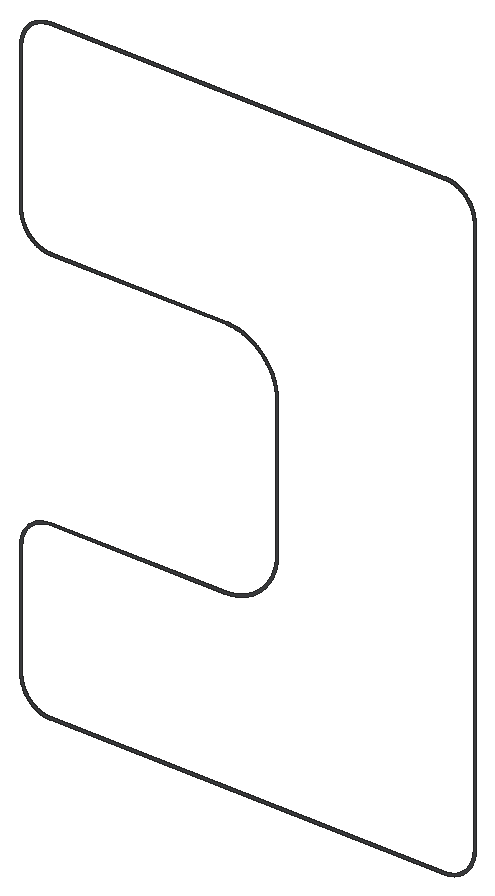
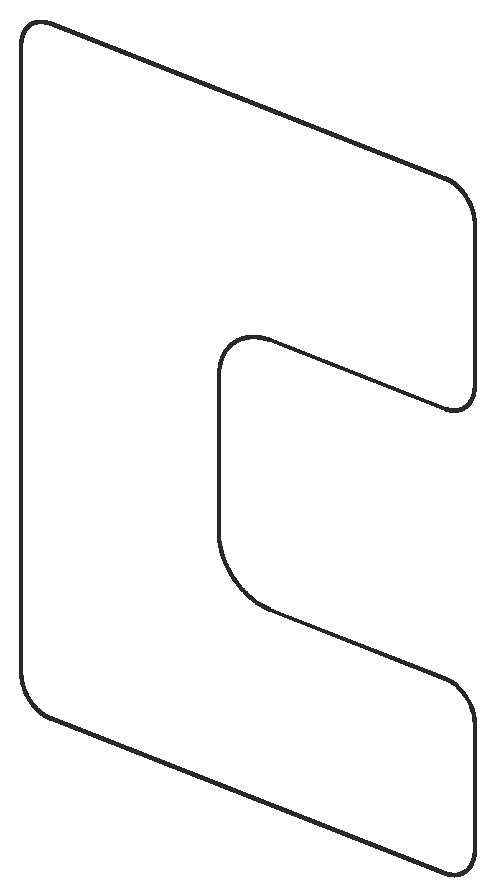
# SketchUp Ruby script. Lengths in inches.
U = 1.inch
M = Sketchup.active_model
def pt(a) = Geom::Point3d.new(a.map { |v| v * U })
def face(e, loops, mat)
  f = e.add_face(loops[0].map { |a| pt(a) })
  loops[1..].each { |l| e.add_face(l.map { |a| pt(a) }).erase! }
  f.material = f.back_material = mat if mat
  f
end
# faces: each face lists its corners as indices into pts; further lists are holes
def faces(e, pts, list, mat = nil) = list.each { |f| face(e, (f[0].is_a?(Array) ? f : [f]).map { |l| l.map { |i| pts[i] } }, mat) }
# xy, xz, yz: faces in a plane at the given z, y or x. An outline is a flat list of corners, or four numbers for a rectangle; further outlines are holes
def ring(l) = l.size == 4 ? [[l[0], l[1]], [l[2], l[1]], [l[2], l[3]], [l[0], l[3]]] : l.each_slice(2).to_a
def flat(e, list, mat, &to3) = list.each { |f| face(e, (f[0].is_a?(Array) ? f : [f]).map { |l| ring(l).map { |u, v| to3.(u, v) } }, mat) }
def xy(e, z, list, mat = nil) = flat(e, list, mat) { |x, y| [x, y, z] }
def xz(e, y, list, mat = nil) = flat(e, list, mat) { |x, z| [x, y, z] }
def yz(e, x, list, mat = nil) = flat(e, list, mat) { |y, z| [x, y, z] }
def lines(e, pts, list) = list.each { |a, b| e.add_line(pt(pts[a]), pt(pts[b])) }
# prism: a flat outline (further loops are holes) pulled along v
def prism(e, loops, v, mat = nil)
  f = face(e, loops, mat); d = Geom::Vector3d.new(v.map { |x| x * U })
  f.pushpull(f.normal.samedirection?(d) ? d.length : -d.length)
end
def box(e, o, s, mat = nil) = prism(e, [[o, [o[0] + s[0], o[1], o[2]], [o[0] + s[0], o[1] + s[1], o[2]], [o[0], o[1] + s[1], o[2]]]], [0, 0, s[2]], mat)
def at(x, y, z, deg = 0) = Geom::Transformation.translation(pt([x, y, z])) * Geom::Transformation.rotation(ORIGIN, Z_AXIS, deg.degrees)
def axes(o, x, y, z) = Geom::Transformation.new([*x, 0, *y, 0, *z, 0, *pt(o).to_a, 1])
def part(name) = M.definitions.add(name)
# library, detail: a bought-in or finely detailed component or shape, given as its bounding box
def library(name, o, s) = part(name).tap { |d| box(d.entities, o, s) }
def detail(e, o, s) = box(e.add_group.entities, o, s)
def put(e, d, t, mat = nil) = e.add_instance(d, t).tap { |i| i.material = mat if mat }
def group(e, t, mat = nil) = e.add_group.tap { |g| g.transformation = t; g.material = mat if mat }.entities
root = M.entities
M.materials.add("1432 AP 8245 TAR ROAD").color = [71, 72, 75]
xz(root,96.87,[[[278.68,171.29,537.32,171.29,537.48,171.3,537.64,171.3,537.8,171.31,537.97,171.31,538.125,171.32,538.29,171.33,538.45,171.34,538.61,171.36,538.93,171.38,539.25,171.42,539.41,171.43,539.73,171.47,539.89,171.5,540.21,171.54,540.37,171.57,540.52,171.6,540.68,171.625,540.84,171.66,541,171.6875,541.16,171.72,541.31,171.75,541.47,171.79,541.63,171.82,541.79,171.86,541.94,171.9,542.1,171.9375,542.25,171.98,542.41,172.02,542.56,172.0625,542.72,172.11,542.875,172.15,543.03,172.2,543.33,172.3,543.49,172.35,543.94,172.5,544.1,172.56,544.25,172.62,544.4,172.67,544.85,172.85,544.99,172.91,545.14,172.98,545.29,173.04,545.4375,173.11,545.58,173.18,545.73,173.24,545.875,173.3125,546.02,173.38,546.16,173.45,546.31,173.53,546.59,173.67,546.73,173.75,547.02,173.91,547.44,174.15,547.57,174.23,547.71,174.3125,547.85,174.4,547.98,174.48,548.12,174.57,548.25,174.66,548.39,174.75,548.52,174.84,548.66,174.93,548.92,175.11,549.05,175.21,549.18,175.3,549.31,175.4,549.4375,175.5,549.56,175.59,549.82,175.79,549.94,175.89,550.07,176,550.19,176.1,550.3125,176.2,550.4375,176.31,550.56,176.41,550.92,176.74,551.03,176.85,551.27,177.07,551.61,177.41,551.72,177.53,551.83,177.64,551.94,177.76,552.05,177.875,552.16,178,552.27,178.11,552.38,178.24,552.48,178.36,552.59,178.48,552.69,178.6,552.8,178.72,552.9,178.85,553,178.97,553.3,179.36,553.39,179.48,553.49,179.61,553.58,179.74,553.68,179.875,553.77,180,553.86,180.14,553.96,180.27,554.05,180.4,554.13,180.54,554.22,180.67,554.31,180.81,554.39,180.94,554.48,181.08,554.5625,181.22,554.65,181.36,554.89,181.78,554.96,181.92,555.12,182.2,555.19,182.34,555.27,182.49,555.41,182.77,555.48,182.92,555.55,183.0625,555.62,183.21,555.68,183.36,555.75,183.5,555.8125,183.65,555.88,183.8,556.18,184.55,556.23,184.7,556.29,184.85,556.39,185.15,556.45,185.3,556.5,185.46,556.55,185.61,556.59,185.76,556.64,185.92,556.6875,186.07,556.73,186.23,556.77,186.38,556.82,186.54,556.86,186.69,556.9,186.85,556.93,187.01,556.97,187.16,557.01,187.32,557.04,187.48,557.07,187.63,557.11,187.79,557.17,188.11,557.19,188.27,557.25,188.59,557.27,188.74,557.3,188.9,557.32,189.0625,557.34,189.22,557.36,189.38,557.39,189.7,557.41,189.86,557.42,190.02,557.4375,190.18,557.45,190.34,557.46,190.5,557.47,190.67,557.48,190.83,557.48,190.99,557.49,191.15,557.49,191.31,557.5,191.47,557.5,561.11,557.49,561.28,557.49,561.4375,557.48,561.6,557.48,561.76,557.45,562.24,557.4375,562.4,557.42,562.5625,557.41,562.72,557.39,562.88,557.36,563.2,557.3,563.68,557.27,563.84,557.25,564,557.19,564.32,557.17,564.48,557.14,564.63,557.11,564.79,557.07,564.95,557.04,565.11,557.01,565.26,556.93,565.58,556.9,565.73,556.82,566.05,556.77,566.2,556.73,566.36,556.6875,566.51,556.64,566.67,556.59,566.82,556.55,566.97,556.45,567.28,556.39,567.43,556.34,567.58,556.29,567.74,556.23,567.89,556.18,568.04,556.12,568.1875,556.06,568.34,555.88,568.79,555.8125,568.93,555.75,569.08,555.68,569.23,555.62,569.375,555.55,569.52,555.48,569.67,555.41,569.8125,555.34,569.96,555.27,570.1,555.19,570.24,555.12,570.38,555.04,570.53,554.96,570.67,554.89,570.81,554.65,571.23,554.5625,571.37,554.48,571.5,554.39,571.64,554.31,571.78,554.22,571.91,554.13,572.05,554.05,572.18,553.96,572.31,553.86,572.45,553.68,572.71,553.58,572.84,553.49,572.97,553.39,573.1,553.3,573.23,553.2,573.36,553.1,573.48,553,573.61,552.9,573.73,552.8,573.86,552.69,573.98,552.59,574.11,552.48,574.23,552.38,574.35,551.94,574.83,551.83,574.94,551.72,575.06,551.61,575.17,551.5,575.29,551.38,575.4,551.27,575.51,551.03,575.74,550.92,575.85,550.8,575.95,550.68,576.0625,550.56,576.17,550.4375,576.28,550.3125,576.38,550.19,576.48,550.07,576.59,549.94,576.69,549.82,576.79,549.56,576.99,549.4375,577.09,549.31,577.1875,549.18,577.28,548.92,577.47,548.79,577.5625,548.66,577.66,548.52,577.75,548.39,577.84,548.25,577.93,548.12,578.01,547.98,578.1,547.85,578.1875,547.71,578.27,547.57,578.35,547.44,578.4375,547.3,578.52,547.02,578.68,546.875,578.76,546.73,578.83,546.59,578.91,546.45,578.98,546.31,579.06,546.16,579.13,546.02,579.2,545.73,579.34,545.58,579.41,545.4375,579.48,545.29,579.54,545.14,579.61,544.99,579.67,544.85,579.73,544.25,579.97,544.1,580.02,543.94,580.08,543.79,580.13,543.64,580.1875,543.49,580.24,543.33,580.29,543.03,580.39,542.875,580.43,542.72,580.48,542.56,580.52,542.41,580.57,542.25,580.61,542.1,580.65,541.94,580.6875,541.79,580.73,541.63,580.76,541.47,580.8,541.31,580.83,541.16,580.87,540.52,580.99,540.37,581.01,540.21,581.04,540.05,581.0625,539.89,581.09,539.09,581.19,538.93,581.2,538.77,581.22,538.29,581.25,538.125,581.26,537.97,581.27,537.8,581.28,537.64,581.28,537.48,581.29,278.52,581.29,278.36,581.28,278.2,581.28,278.03,581.27,277.875,581.26,277.71,581.25,277.23,581.22,277.07,581.2,276.91,581.19,276.11,581.09,275.95,581.0625,275.79,581.04,275.63,581.01,275.48,580.99,274.84,580.87,274.69,580.83,274.53,580.8,274.37,580.76,274.21,580.73,274.06,580.6875,273.9,580.65,273.75,580.61,273.59,580.57,273.44,580.52,273.28,580.48,273.125,580.43,272.97,580.39,272.67,580.29,272.51,580.24,272.36,580.1875,272.21,580.13,272.06,580.08,271.9,580.02,271.75,579.97,271.15,579.73,271.01,579.67,270.86,579.61,270.71,579.54,270.5625,579.48,270.42,579.41,270.27,579.34,269.98,579.2,269.84,579.13,269.69,579.06,269.55,578.98,269.41,578.91,269.27,578.83,269.125,578.76,268.98,578.68,268.7,578.52,268.56,578.4375,268.43,578.35,268.29,578.27,268.15,578.1875,268.02,578.1,267.88,578.01,267.75,577.93,267.61,577.84,267.48,577.75,267.34,577.66,267.21,577.5625,267.08,577.47,266.82,577.28,266.69,577.1875,266.5625,577.09,266.44,576.99,266.18,576.79,266.06,576.69,265.93,576.59,265.81,576.48,265.6875,576.38,265.5625,576.28,265.44,576.17,265.32,576.0625,265.2,575.95,265.08,575.85,264.97,575.74,264.73,575.51,264.62,575.4,264.5,575.29,264.39,575.17,264.28,575.06,264.17,574.94,264.06,574.83,263.62,574.35,263.52,574.23,263.41,574.11,263.31,573.98,263.2,573.86,263.1,573.73,263,573.61,262.9,573.48,262.8,573.36,262.7,573.23,262.61,573.1,262.51,572.97,262.42,572.84,262.32,572.71,262.14,572.45,262.04,572.31,261.95,572.18,261.87,572.05,261.78,571.91,261.69,571.78,261.61,571.64,261.52,571.5,261.4375,571.37,261.35,571.23,261.11,570.81,261.04,570.67,260.96,570.53,260.88,570.38,260.81,570.24,260.73,570.1,260.66,569.96,260.59,569.8125,260.52,569.67,260.45,569.52,260.38,569.375,260.32,569.23,260.25,569.08,260.1875,568.93,260.12,568.79,259.94,568.34,259.88,568.1875,259.82,568.04,259.77,567.89,259.71,567.74,259.66,567.58,259.61,567.43,259.55,567.28,259.45,566.97,259.41,566.82,259.36,566.67,259.3125,566.51,259.27,566.36,259.23,566.2,259.18,566.05,259.1,565.73,259.07,565.58,258.99,565.26,258.96,565.11,258.93,564.95,258.89,564.79,258.86,564.63,258.83,564.48,258.81,564.32,258.75,564,258.73,563.84,258.7,563.68,258.64,563.2,258.61,562.88,258.59,562.72,258.58,562.5625,258.5625,562.4,258.55,562.24,258.52,561.76,258.52,561.6,258.51,561.4375,258.51,561.28,258.5,561.11,258.5,464.47,258.51,464.31,258.51,464.15,258.52,463.99,258.52,463.83,258.53,463.67,258.54,463.5,258.55,463.34,258.5625,463.18,258.58,463.02,258.59,462.86,258.61,462.7,258.64,462.38,258.66,462.22,258.68,462.0625,258.7,461.9,258.73,461.74,258.75,461.59,258.81,461.27,258.83,461.11,258.89,460.79,258.93,460.63,258.96,460.48,258.99,460.32,259.03,460.16,259.07,460.01,259.1,459.85,259.14,459.69,259.18,459.54,259.23,459.38,259.27,459.23,259.3125,459.07,259.36,458.92,259.41,458.76,259.45,458.61,259.5,458.46,259.55,458.3,259.61,458.15,259.71,457.85,259.77,457.7,259.82,457.55,260.12,456.8,260.1875,456.65,260.25,456.5,260.32,456.36,260.38,456.21,260.45,456.0625,260.52,455.92,260.59,455.77,260.73,455.49,260.81,455.34,260.88,455.2,261.04,454.92,261.11,454.78,261.35,454.36,261.4375,454.22,261.52,454.08,261.61,453.94,261.69,453.81,261.78,453.67,261.87,453.54,261.95,453.4,262.04,453.27,262.14,453.14,262.23,453,262.32,452.875,262.42,452.74,262.51,452.61,262.61,452.48,262.7,452.36,263,451.97,263.1,451.85,263.2,451.72,263.31,451.6,263.41,451.48,263.52,451.36,263.62,451.24,263.73,451.11,263.84,451,263.95,450.875,264.06,450.76,264.17,450.64,264.28,450.53,264.39,450.41,264.73,450.07,264.97,449.85,265.08,449.74,265.44,449.41,265.5625,449.31,265.6875,449.2,265.81,449.1,265.93,449,266.06,448.89,266.18,448.79,266.44,448.59,266.5625,448.5,266.69,448.4,266.82,448.3,266.95,448.21,267.08,448.11,267.34,447.93,267.48,447.84,267.61,447.75,267.75,447.66,267.88,447.57,268.02,447.48,268.15,447.4,268.29,447.3125,268.43,447.23,268.56,447.15,268.98,446.91,269.27,446.75,269.41,446.67,269.69,446.53,269.84,446.45,269.98,446.38,270.125,446.3125,270.27,446.24,270.42,446.18,270.5625,446.11,270.71,446.04,270.86,445.98,271.01,445.91,271.15,445.85,271.6,445.67,271.75,445.62,271.9,445.56,272.06,445.5,272.51,445.35,272.67,445.3,272.97,445.2,273.125,445.15,273.28,445.11,273.44,445.0625,273.59,445.02,273.75,444.98,273.9,444.9375,274.06,444.9,274.21,444.86,274.37,444.82,274.53,444.79,274.69,444.75,274.84,444.72,275,444.6875,275.16,444.66,275.32,444.625,275.48,444.6,275.63,444.57,275.79,444.54,276.11,444.5,276.27,444.47,276.59,444.43,276.75,444.42,277.07,444.38,277.39,444.36,277.55,444.34,277.71,444.33,277.875,444.32,278.03,444.31,278.2,444.31,278.36,444.3,278.52,444.3,278.68,444.29,393.4375,444.29,393.875,444.28,394.32,444.27,394.75,444.25,395.19,444.22,395.63,444.1875,396.07,444.15,396.5,444.11,396.9375,444.06,397.37,444.01,397.81,443.95,398.67,443.81,399.1,443.73,399.54,443.65,399.97,443.56,400.39,443.47,400.82,443.37,401.25,443.26,401.67,443.15,402.93,442.79,403.77,442.51,404.18,442.37,404.59,442.22,405.01,442.07,405.41,441.91,405.82,441.74,406.22,441.57,406.625,441.4,407.03,441.21,407.42,441.03,407.82,440.84,408.21,440.64,408.6,440.4375,408.98,440.23,409.37,440.02,410.13,439.58,410.5,439.36,411.25,438.89,411.61,438.65,412.33,438.15,412.69,437.89,413.39,437.37,413.74,437.1,414.08,436.83,414.76,436.27,415.09,435.98,415.42,435.6875,415.74,435.39,416.06,435.09,416.375,434.79,417,434.17,417.9,433.21,418.1875,432.88,418.47,432.55,418.76,432.21,419.03,431.875,419.31,431.53,419.58,431.1875,419.84,430.84,420.1,430.48,420.36,430.125,420.61,429.77,420.85,429.4,421.1,429.04,421.33,428.67,421.5625,428.3,421.79,427.92,422.23,427.16,422.44,426.78,422.65,426.39,423.05,425.61,423.24,425.21,423.42,424.82,423.78,424.02,423.95,423.61,424.12,423.21,424.27,422.8,424.43,422.39,424.58,421.97,424.72,421.56,424.86,421.14,424.99,420.73,425.12,420.31,425.24,419.89,425.36,419.46,425.47,419.04,425.57,418.61,425.67,418.19,425.77,417.76,425.86,417.33,425.9375,416.9,426.02,416.47,426.09,416.03,426.15,415.6,426.21,415.16,426.27,414.73,426.32,414.29,426.36,413.86,426.4,413.42,426.43,412.98,426.45,412.55,426.49,411.67,426.5,411.23,426.5,320.35,426.49,319.92,426.43,318.6,426.4,318.16,426.36,317.73,426.32,317.29,426.27,316.85,426.15,315.99,426.09,315.55,426.02,315.12,425.9375,314.6875,425.86,314.26,425.77,313.83,425.57,312.97,425.47,312.55,425.36,312.12,425.12,311.28,424.86,310.44,424.72,310.02,424.58,309.61,424.43,309.2,424.27,308.79,424.12,308.38,423.95,307.97,423.78,307.57,423.24,306.37,423.05,305.98,422.85,305.58,422.65,305.19,422.44,304.81,422.23,304.42,421.79,303.66,421.5625,303.29,421.33,302.92,421.1,302.55,420.85,302.18,420.61,301.82,420.36,301.46,420.1,301.1,419.58,300.4,419.31,300.05,419.03,299.71,418.76,299.37,418.47,299.04,418.1875,298.7,417.9,298.375,417.6,298.05,417.3,297.73,417,297.42,416.6875,297.1,416.375,296.8,416.06,296.49,415.74,296.19,415.42,295.9,414.76,295.32,413.74,294.48,413.39,294.21,412.69,293.69,412.33,293.43,411.97,293.18,411.61,292.9375,411.25,292.7,410.875,292.46,410.5,292.23,410.13,292,409.75,291.78,409.37,291.5625,408.98,291.35,408.6,291.14,408.21,290.94,407.82,290.75,407.42,290.56,407.03,290.37,406.625,290.1875,406.22,290.01,405.82,289.84,405.41,289.68,405.01,289.52,404.59,289.36,404.18,289.21,403.77,289.07,403.35,288.93,402.51,288.67,401.67,288.43,401.25,288.32,400.39,288.12,399.97,288.02,399.54,287.9375,399.1,287.85,398.67,287.78,398.24,287.7,397.81,287.64,397.37,287.58,396.9375,287.52,396.5,287.48,396.07,287.43,395.63,287.4,395.19,287.36,394.75,287.34,394.32,287.32,393.875,287.3,393.4375,287.29,279,287.29,276.32,287.12,273.69,286.59,271.15,285.73,268.75,284.55,266.52,283.06,264.5,281.29,262.74,279.27,261.25,277.04,260.06,274.64,259.2,272.1,258.68,269.47,258.5,266.79,258.5,191.47,258.51,191.31,258.51,191.15,258.52,190.99,258.52,190.83,258.53,190.67,258.54,190.5,258.55,190.34,258.5625,190.18,258.58,190.02,258.59,189.86,258.61,189.7,258.64,189.38,258.66,189.22,258.68,189.0625,258.7,188.9,258.73,188.74,258.75,188.59,258.81,188.27,258.83,188.11,258.89,187.79,258.93,187.63,258.96,187.48,258.99,187.32,259.03,187.16,259.07,187.01,259.1,186.85,259.14,186.69,259.18,186.54,259.23,186.38,259.27,186.23,259.3125,186.07,259.36,185.92,259.41,185.76,259.45,185.61,259.5,185.46,259.55,185.3,259.61,185.15,259.71,184.85,259.77,184.7,259.82,184.55,260.12,183.8,260.1875,183.65,260.25,183.5,260.32,183.36,260.38,183.21,260.45,183.0625,260.52,182.92,260.59,182.77,260.73,182.49,260.81,182.34,260.88,182.2,261.04,181.92,261.11,181.78,261.35,181.36,261.4375,181.22,261.52,181.08,261.61,180.94,261.69,180.81,261.78,180.67,261.87,180.54,261.95,180.4,262.04,180.27,262.14,180.14,262.23,180,262.32,179.875,262.42,179.74,262.51,179.61,262.61,179.48,262.7,179.36,263,178.97,263.1,178.85,263.2,178.72,263.31,178.6,263.41,178.48,263.52,178.36,263.62,178.24,263.73,178.11,263.84,178,263.95,177.875,264.06,177.76,264.17,177.64,264.28,177.53,264.39,177.41,264.73,177.07,264.97,176.85,265.08,176.74,265.44,176.41,265.5625,176.31,265.6875,176.2,265.81,176.1,265.93,176,266.06,175.89,266.18,175.79,266.44,175.59,266.5625,175.5,266.69,175.4,266.82,175.3,266.95,175.21,267.08,175.11,267.34,174.93,267.48,174.84,267.61,174.75,267.75,174.66,267.88,174.57,268.02,174.48,268.15,174.4,268.29,174.3125,268.43,174.23,268.56,174.15,268.98,173.91,269.27,173.75,269.41,173.67,269.69,173.53,269.84,173.45,269.98,173.38,270.125,173.3125,270.27,173.24,270.42,173.18,270.5625,173.11,270.71,173.04,270.86,172.98,271.01,172.91,271.15,172.85,271.6,172.67,271.75,172.62,271.9,172.56,272.06,172.5,272.51,172.35,272.67,172.3,272.97,172.2,273.125,172.15,273.28,172.11,273.44,172.0625,273.59,172.02,273.75,171.98,273.9,171.9375,274.06,171.9,274.21,171.86,274.37,171.82,274.53,171.79,274.69,171.75,274.84,171.72,275,171.6875,275.16,171.66,275.32,171.625,275.48,171.6,275.63,171.57,275.79,171.54,276.11,171.5,276.27,171.47,276.59,171.43,276.75,171.42,277.07,171.38,277.39,171.36,277.55,171.34,277.71,171.33,277.875,171.32,278.03,171.31,278.2,171.31,278.36,171.3,278.52,171.3],[278.7,172.79,278.55,172.8,278.4,172.8,278.25,172.81,278.1,172.8125,277.96,172.82,277.36,172.86,277.21,172.875,277.0625,172.89,276.92,172.91,276.77,172.92,276.32,172.98,276.18,173,276.03,173.03,275.73,173.07,275.59,173.1,275.29,173.16,275.15,173.1875,275,173.22,274.86,173.25,274.71,173.28,274.56,173.32,274.42,173.35,274.27,173.39,273.99,173.47,273.84,173.51,273.56,173.59,273.41,173.63,273.27,173.68,273.13,173.72,272.85,173.82,272.7,173.87,272.5625,173.92,272.42,173.97,272.14,174.07,272.01,174.125,271.87,174.18,271.59,174.3,271.45,174.35,271.32,174.41,271.18,174.48,271.05,174.54,270.91,174.6,270.78,174.66,270.64,174.73,270.51,174.8,270.375,174.86,270.24,174.93,269.72,175.21,269.59,175.29,269.46,175.36,269.33,175.4375,269.2,175.51,269.07,175.59,268.95,175.67,268.69,175.83,268.57,175.91,268.44,175.99,268.32,176.08,268.2,176.16,268.07,176.25,267.95,176.33,267.59,176.6,267.47,176.6875,267.35,176.78,267.24,176.87,267.12,176.96,267,177.06,266.89,177.15,266.77,177.25,266.66,177.34,266.44,177.54,266.32,177.64,265.99,177.94,265.78,178.15,265.67,178.25,265.46,178.46,265.36,178.57,265.25,178.68,265.15,178.79,265.05,178.89,264.95,179,264.85,179.12,264.55,179.45,264.46,179.57,264.36,179.68,264.27,179.8,264.17,179.91,263.9,180.27,263.81,180.38,263.72,180.5,263.54,180.75,263.46,180.87,263.37,180.99,263.29,181.11,263.2,181.24,263.12,181.36,263.04,181.49,262.96,181.61,262.88,181.74,262.8,181.86,262.72,181.99,262.65,182.12,262.57,182.25,262.5,182.38,262.42,182.51,262.14,183.03,262.07,183.17,262,183.3,261.9375,183.43,261.87,183.57,261.81,183.7,261.75,183.84,261.68,183.97,261.62,184.11,261.5625,184.25,261.5,184.38,261.45,184.52,261.33,184.8,261.28,184.9375,261.23,185.08,261.17,185.22,261.125,185.36,261.07,185.5,261.02,185.64,260.98,185.78,260.93,185.92,260.88,186.0625,260.84,186.21,260.8,186.35,260.75,186.49,260.71,186.63,260.67,186.78,260.63,186.92,260.6,187.07,260.56,187.21,260.52,187.36,260.49,187.5,260.46,187.65,260.43,187.79,260.39,187.9375,260.37,188.09,260.34,188.23,260.28,188.53,260.26,188.67,260.23,188.82,260.21,188.97,260.19,189.11,260.11,189.71,260.1,189.86,260.08,190,260.01,191.05,260.01,191.34,260,191.49,260,266.79,260.16,269.27,260.65,271.71,261.45,274.0625,262.55,276.29,263.93,278.36,265.56,280.23,267.43,281.87,269.5,283.25,271.73,284.35,274.08,285.14,276.52,285.63,279,285.79,393,285.79,393.46,285.8,393.92,285.8,394.83,285.84,395.75,285.9,396.2,285.9375,396.66,285.98,397.11,286.03,397.57,286.09,398.02,286.15,398.48,286.22,399.83,286.46,400.28,286.56,400.72,286.66,401.17,286.76,401.62,286.87,402.06,286.98,402.5,287.11,402.94,287.23,403.82,287.51,404.25,287.65,404.68,287.8,405.97,288.28,406.39,288.46,406.82,288.63,407.24,288.82,407.65,289.01,408.07,289.2,408.48,289.4,409.3,289.82,409.7,290.03,410.1,290.25,410.9,290.71,411.68,291.19,412.0625,291.4375,412.44,291.69,413.2,292.21,414.31,293.02,414.67,293.31,415.03,293.59,415.38,293.88,416.08,294.48,416.42,294.78,416.76,295.09,417.09,295.4,417.75,296.04,418.39,296.7,418.7,297.03,419.01,297.37,419.3125,297.71,419.61,298.0625,419.91,298.41,420.2,298.77,420.49,299.125,420.77,299.49,421.04,299.85,421.32,300.22,421.58,300.59,422.1,301.35,422.35,301.73,422.6,302.12,422.84,302.5,423.08,302.9,423.3125,303.29,423.54,303.69,423.76,304.09,423.97,304.5,424.19,304.9,424.39,305.3125,424.59,305.72,424.79,306.14,424.97,306.56,425.16,306.98,425.34,307.4,425.51,307.82,425.68,308.25,425.84,308.68,426.14,309.54,426.29,309.98,426.43,310.41,426.56,310.85,426.6875,311.29,426.81,311.73,426.92,312.18,427.03,312.62,427.14,313.07,427.24,313.52,427.33,313.96,427.49,314.86,427.57,315.32,427.64,315.77,427.7,316.22,427.76,316.68,427.81,317.13,427.89,318.05,427.93,318.5,427.97,319.42,427.99,319.875,428,320.33,428,411.25,427.99,411.71,427.97,412.17,427.93,413.08,427.89,413.54,427.85,413.99,427.81,414.45,427.76,414.91,427.7,415.36,427.64,415.8125,427.57,416.27,427.33,417.62,427.24,418.07,427.14,418.52,427.03,418.96,426.92,419.41,426.81,419.85,426.6875,420.29,426.56,420.73,426.43,421.17,426.29,421.61,426.14,422.04,425.99,422.48,425.84,422.91,425.68,423.33,425.51,423.76,425.34,424.1875,425.16,424.61,424.97,425.03,424.79,425.45,424.19,426.68,423.97,427.09,423.76,427.49,423.54,427.89,423.3125,428.29,423.08,428.6875,422.84,429.08,422.6,429.47,422.35,429.85,422.1,430.24,421.84,430.62,421.32,431.36,421.04,431.73,420.77,432.1,420.49,432.46,420.2,432.82,419.91,433.17,419.61,433.52,419.3125,433.87,419.01,434.21,418.7,434.55,418.39,434.88,417.75,435.54,417.09,436.18,416.76,436.49,416.08,437.11,415.73,437.41,415.03,437.99,414.67,438.28,414.31,438.56,413.94,438.84,413.57,439.11,413.2,439.375,412.82,439.64,412.44,439.89,412.0625,440.15,411.68,440.39,410.9,440.87,410.1,441.33,409.3,441.77,408.89,441.98,408.07,442.38,407.65,442.58,407.24,442.77,406.82,442.95,406.39,443.13,405.97,443.3,405.54,443.47,405.11,443.63,403.82,444.08,403.38,444.22,402.5,444.48,401.62,444.72,401.17,444.82,400.72,444.93,400.28,445.03,399.38,445.21,398.93,445.29,398.48,445.36,398.02,445.43,397.57,445.49,397.11,445.55,396.66,445.6,396.2,445.65,395.75,445.68,395.29,445.72,394.83,445.74,394.375,445.77,393.92,445.78,393.46,445.79,278.7,445.79,278.55,445.8,278.4,445.8,278.25,445.81,278.1,445.8125,277.96,445.82,277.36,445.86,277.21,445.875,277.0625,445.89,276.92,445.91,276.77,445.92,276.32,445.98,276.18,446,276.03,446.03,275.73,446.07,275.59,446.1,275.29,446.16,275.15,446.1875,275,446.22,274.86,446.25,274.71,446.28,274.56,446.32,274.42,446.35,274.27,446.39,273.99,446.47,273.84,446.51,273.56,446.59,273.41,446.63,273.27,446.68,273.13,446.72,272.85,446.82,272.7,446.87,272.5625,446.92,272.42,446.97,272.14,447.07,272.01,447.125,271.87,447.18,271.59,447.3,271.45,447.35,271.32,447.41,271.18,447.48,271.05,447.54,270.91,447.6,270.78,447.66,270.64,447.73,270.51,447.8,270.375,447.86,270.24,447.93,269.72,448.21,269.59,448.29,269.46,448.36,269.33,448.4375,269.2,448.51,269.07,448.59,268.95,448.67,268.69,448.83,268.57,448.91,268.44,448.99,268.32,449.08,268.2,449.16,268.07,449.25,267.95,449.33,267.59,449.6,267.47,449.6875,267.35,449.78,267.24,449.87,267.12,449.96,267,450.06,266.89,450.15,266.77,450.25,266.66,450.34,266.44,450.54,266.32,450.64,265.99,450.94,265.78,451.15,265.67,451.25,265.46,451.46,265.36,451.57,265.25,451.68,265.15,451.79,265.05,451.89,264.95,452,264.85,452.12,264.55,452.45,264.46,452.57,264.36,452.68,264.27,452.8,264.17,452.91,263.9,453.27,263.81,453.38,263.72,453.5,263.54,453.75,263.46,453.87,263.37,453.99,263.29,454.11,263.2,454.24,263.12,454.36,263.04,454.49,262.96,454.61,262.88,454.74,262.8,454.86,262.72,454.99,262.65,455.12,262.57,455.25,262.5,455.38,262.42,455.51,262.14,456.03,262.07,456.17,262,456.3,261.9375,456.43,261.87,456.57,261.81,456.7,261.75,456.84,261.68,456.97,261.62,457.11,261.5625,457.25,261.5,457.38,261.45,457.52,261.33,457.8,261.28,457.9375,261.23,458.08,261.17,458.22,261.125,458.36,261.07,458.5,261.02,458.64,260.98,458.78,260.93,458.92,260.88,459.0625,260.84,459.21,260.8,459.35,260.75,459.49,260.71,459.63,260.67,459.78,260.63,459.92,260.6,460.07,260.56,460.21,260.52,460.36,260.49,460.5,260.46,460.65,260.43,460.79,260.39,460.9375,260.37,461.09,260.34,461.23,260.28,461.53,260.26,461.67,260.23,461.82,260.21,461.97,260.19,462.11,260.11,462.71,260.1,462.86,260.08,463,260.01,464.05,260.01,464.34,260,464.49,260,561.09,260.01,561.24,260.01,561.54,260.02,561.6875,260.03,561.84,260.04,561.99,260.05,562.13,260.08,562.58,260.1,562.73,260.11,562.88,260.13,563.03,260.15,563.17,260.21,563.62,260.23,563.76,260.26,563.91,260.28,564.06,260.31,564.21,260.34,564.35,260.37,564.5,260.39,564.65,260.43,564.79,260.46,564.9375,260.49,565.08,260.52,565.23,260.56,565.37,260.6,565.52,260.63,565.66,260.67,565.81,260.75,566.09,260.8,566.24,260.88,566.52,260.93,566.66,260.98,566.81,261.02,566.95,261.07,567.09,261.125,567.23,261.17,567.37,261.23,567.51,261.33,567.79,261.39,567.92,261.45,568.0625,261.5,568.2,261.5625,568.34,261.62,568.47,261.68,568.61,261.75,568.75,261.81,568.88,261.87,569.02,261.9375,569.15,262,569.28,262.07,569.42,262.21,569.68,262.28,569.8125,262.35,569.95,262.42,570.08,262.5,570.21,262.57,570.34,262.65,570.46,262.72,570.59,262.88,570.85,262.96,570.97,263.04,571.1,263.12,571.22,263.2,571.35,263.29,571.47,263.37,571.59,263.46,571.72,263.54,571.84,263.9,572.32,263.99,572.4375,264.08,572.55,264.17,572.67,264.27,572.79,264.36,572.9,264.46,573.02,264.55,573.13,264.65,573.24,264.75,573.36,264.95,573.58,265.05,573.6875,265.15,573.8,265.25,573.91,265.36,574.01,265.56,574.23,265.67,574.33,265.78,574.4375,265.89,574.54,265.99,574.64,266.1,574.74,266.21,574.85,266.32,574.95,266.44,575.04,266.77,575.34,266.89,575.43,267,575.53,267.24,575.71,267.35,575.8,267.47,575.9,267.71,576.08,267.83,576.16,268.07,576.34,268.2,576.42,268.32,576.51,268.44,576.59,268.57,576.67,268.69,576.75,268.95,576.91,269.07,576.99,269.33,577.15,269.46,577.22,269.59,577.3,270.24,577.65,270.51,577.79,270.64,577.85,270.78,577.92,270.91,577.98,271.05,578.05,271.18,578.11,271.32,578.17,271.45,578.23,271.73,578.35,271.87,578.4,272.01,578.46,272.14,578.51,272.28,578.57,272.42,578.62,272.5625,578.67,272.7,578.72,272.85,578.77,272.99,578.82,273.13,578.86,273.27,578.91,273.41,578.95,273.56,579,273.84,579.08,273.99,579.12,274.27,579.2,274.42,579.23,274.56,579.27,274.86,579.33,275,579.37,275.15,579.4,275.29,579.43,275.44,579.46,275.59,579.48,275.73,579.51,275.88,579.53,276.03,579.56,276.18,579.58,276.32,579.6,276.92,579.68,277.0625,579.69,277.21,579.71,277.96,579.76,278.1,579.77,278.25,579.78,278.4,579.78,278.55,579.79,537.45,579.79,537.6,579.78,537.75,579.78,537.9,579.77,538.04,579.76,538.79,579.71,538.9375,579.69,539.08,579.68,539.68,579.6,539.82,579.58,539.97,579.56,540.12,579.53,540.27,579.51,540.41,579.48,540.56,579.46,540.71,579.43,540.85,579.4,541,579.37,541.14,579.33,541.44,579.27,541.58,579.23,541.73,579.2,542.01,579.12,542.16,579.08,542.44,579,542.59,578.95,542.73,578.91,542.87,578.86,543.01,578.82,543.15,578.77,543.3,578.72,543.4375,578.67,543.58,578.62,543.72,578.57,543.86,578.51,543.99,578.46,544.13,578.4,544.27,578.35,544.55,578.23,544.68,578.17,544.82,578.11,544.95,578.05,545.09,577.98,545.22,577.92,545.36,577.85,545.49,577.79,545.76,577.65,546.41,577.3,546.54,577.22,546.67,577.15,546.93,576.99,547.05,576.91,547.31,576.75,547.43,576.67,547.56,576.59,547.68,576.51,547.8,576.42,547.93,576.34,548.17,576.16,548.29,576.08,548.53,575.9,548.65,575.8,548.76,575.71,549,575.53,549.11,575.43,549.23,575.34,549.56,575.04,549.68,574.95,549.79,574.85,549.9,574.74,550.01,574.64,550.11,574.54,550.22,574.4375,550.33,574.33,550.44,574.23,550.64,574.01,550.75,573.91,550.85,573.8,550.95,573.6875,551.05,573.58,551.25,573.36,551.35,573.24,551.45,573.13,551.54,573.02,551.64,572.9,551.73,572.79,551.83,572.67,551.92,572.55,552.01,572.4375,552.1,572.32,552.46,571.84,552.54,571.72,552.63,571.59,552.71,571.47,552.8,571.35,552.88,571.22,552.96,571.1,553.04,570.97,553.12,570.85,553.28,570.59,553.35,570.46,553.43,570.34,553.5,570.21,553.58,570.08,553.65,569.95,553.72,569.8125,553.79,569.68,553.93,569.42,554,569.28,554.0625,569.15,554.13,569.02,554.19,568.88,554.25,568.75,554.32,568.61,554.38,568.47,554.4375,568.34,554.5,568.2,554.55,568.0625,554.61,567.92,554.67,567.79,554.77,567.51,554.83,567.37,554.875,567.23,554.93,567.09,554.98,566.95,555.02,566.81,555.07,566.66,555.12,566.52,555.2,566.24,555.25,566.09,555.33,565.81,555.37,565.66,555.4,565.52,555.44,565.37,555.48,565.23,555.51,565.08,555.54,564.9375,555.57,564.79,555.61,564.65,555.63,564.5,555.66,564.35,555.69,564.21,555.72,564.06,555.74,563.91,555.77,563.76,555.79,563.62,555.85,563.17,555.87,563.03,555.89,562.88,555.9,562.73,555.92,562.58,555.95,562.13,555.96,561.99,555.97,561.84,555.98,561.6875,555.99,561.54,555.99,561.24,556,561.09,556,191.49,555.99,191.34,555.99,191.05,555.92,190,555.9,189.86,555.89,189.71,555.81,189.11,555.79,188.97,555.77,188.82,555.74,188.67,555.72,188.53,555.66,188.23,555.63,188.09,555.61,187.9375,555.57,187.79,555.54,187.65,555.51,187.5,555.48,187.36,555.44,187.21,555.4,187.07,555.37,186.92,555.33,186.78,555.29,186.63,555.25,186.49,555.2,186.35,555.16,186.21,555.12,186.0625,555.07,185.92,555.02,185.78,554.98,185.64,554.93,185.5,554.875,185.36,554.83,185.22,554.77,185.08,554.72,184.9375,554.67,184.8,554.55,184.52,554.5,184.38,554.4375,184.25,554.38,184.11,554.32,183.97,554.25,183.84,554.19,183.7,554.13,183.57,554.0625,183.43,554,183.3,553.93,183.17,553.86,183.03,553.58,182.51,553.5,182.38,553.43,182.25,553.35,182.12,553.28,181.99,553.2,181.86,553.12,181.74,553.04,181.61,552.96,181.49,552.88,181.36,552.8,181.24,552.71,181.11,552.63,180.99,552.54,180.87,552.46,180.75,552.28,180.5,552.19,180.38,552.1,180.27,551.83,179.91,551.73,179.8,551.64,179.68,551.54,179.57,551.45,179.45,551.15,179.12,551.05,179,550.95,178.89,550.85,178.79,550.75,178.68,550.64,178.57,550.54,178.46,550.33,178.25,550.22,178.15,550.01,177.94,549.68,177.64,549.56,177.54,549.34,177.34,549.23,177.25,549.11,177.15,549,177.06,548.88,176.96,548.76,176.87,548.65,176.78,548.53,176.6875,548.41,176.6,548.05,176.33,547.93,176.25,547.8,176.16,547.68,176.08,547.56,175.99,547.43,175.91,547.31,175.83,547.05,175.67,546.93,175.59,546.8,175.51,546.67,175.4375,546.54,175.36,546.41,175.29,546.28,175.21,545.76,174.93,545.625,174.86,545.49,174.8,545.36,174.73,545.22,174.66,545.09,174.6,544.95,174.54,544.82,174.48,544.68,174.41,544.55,174.35,544.41,174.3,544.13,174.18,543.99,174.125,543.86,174.07,543.58,173.97,543.4375,173.92,543.3,173.87,543.15,173.82,542.87,173.72,542.73,173.68,542.59,173.63,542.44,173.59,542.16,173.51,542.01,173.47,541.73,173.39,541.58,173.35,541.44,173.32,541.29,173.28,541.14,173.25,541,173.22,540.85,173.1875,540.71,173.16,540.41,173.1,540.27,173.07,539.97,173.03,539.82,173,539.68,172.98,539.23,172.92,539.08,172.91,538.9375,172.89,538.79,172.875,538.64,172.86,538.04,172.82,537.9,172.8125,537.75,172.81,537.6,172.8,537.45,172.8,537.3,172.79]]],"1432 AP 8245 TAR ROAD")
